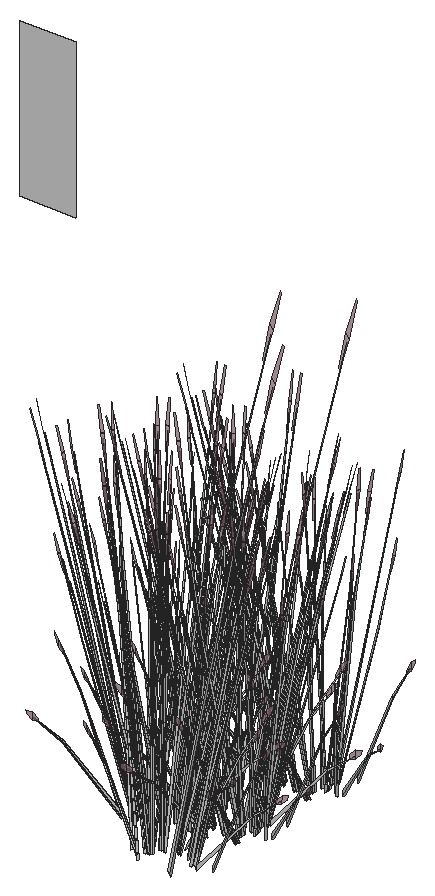
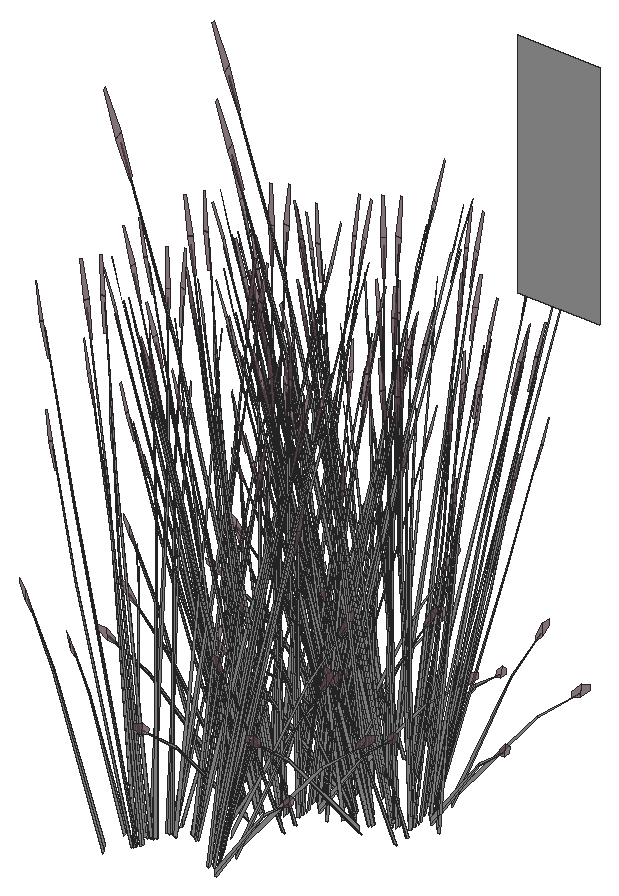
# SketchUp Ruby script. Lengths in inches.
U = 1.inch
M = Sketchup.active_model
def pt(a) = Geom::Point3d.new(a.map { |v| v * U })
def face(e, loops, mat)
  f = e.add_face(loops[0].map { |a| pt(a) })
  loops[1..].each { |l| e.add_face(l.map { |a| pt(a) }).erase! }
  f.material = f.back_material = mat if mat
  f
end
# faces: each face lists its corners as indices into pts; further lists are holes
def faces(e, pts, list, mat = nil) = list.each { |f| face(e, (f[0].is_a?(Array) ? f : [f]).map { |l| l.map { |i| pts[i] } }, mat) }
# xy, xz, yz: faces in a plane at the given z, y or x. An outline is a flat list of corners, or four numbers for a rectangle; further outlines are holes
def ring(l) = l.size == 4 ? [[l[0], l[1]], [l[2], l[1]], [l[2], l[3]], [l[0], l[3]]] : l.each_slice(2).to_a
def flat(e, list, mat, &to3) = list.each { |f| face(e, (f[0].is_a?(Array) ? f : [f]).map { |l| ring(l).map { |u, v| to3.(u, v) } }, mat) }
def xy(e, z, list, mat = nil) = flat(e, list, mat) { |x, y| [x, y, z] }
def xz(e, y, list, mat = nil) = flat(e, list, mat) { |x, z| [x, y, z] }
def yz(e, x, list, mat = nil) = flat(e, list, mat) { |y, z| [x, y, z] }
def lines(e, pts, list) = list.each { |a, b| e.add_line(pt(pts[a]), pt(pts[b])) }
# prism: a flat outline (further loops are holes) pulled along v
def prism(e, loops, v, mat = nil)
  f = face(e, loops, mat); d = Geom::Vector3d.new(v.map { |x| x * U })
  f.pushpull(f.normal.samedirection?(d) ? d.length : -d.length)
end
def box(e, o, s, mat = nil) = prism(e, [[o, [o[0] + s[0], o[1], o[2]], [o[0] + s[0], o[1] + s[1], o[2]], [o[0], o[1] + s[1], o[2]]]], [0, 0, s[2]], mat)
def at(x, y, z, deg = 0) = Geom::Transformation.translation(pt([x, y, z])) * Geom::Transformation.rotation(ORIGIN, Z_AXIS, deg.degrees)
def axes(o, x, y, z) = Geom::Transformation.new([*x, 0, *y, 0, *z, 0, *pt(o).to_a, 1])
def part(name) = M.definitions.add(name)
# library, detail: a bought-in or finely detailed component or shape, given as its bounding box
def library(name, o, s) = part(name).tap { |d| box(d.entities, o, s) }
def detail(e, o, s) = box(e.add_group.entities, o, s)
def put(e, d, t, mat = nil) = e.add_instance(d, t).tap { |i| i.material = mat if mat }
def group(e, t, mat = nil) = e.add_group.tap { |g| g.transformation = t; g.material = mat if mat }.entities
root = M.entities
M.materials.add("LightPink_Translucent").color = [144, 107, 117]
M.materials["LightPink_Translucent"].alpha = 0.75
M.materials.add("[_0053_Ivory_]").color = [200, 200, 200]
c1 = part("blade")
p = [[2.15,0.21,22],[0,0.17,0],[0.09,0.45,0],[2.18,0.31,22],[2.29,0.31,22],[0.38,0.45,0],
  [2.48,0.24,33],[2.49,0.24,33],[2.48,0.22,33]]
faces(c1.entities,p,[[0,1,2,3],[4,5,2,3],[6,3,4,7],[8,0,3,6]])
c2 = part("seeds")
p = [[0.3,-0.1,1.38],[-0.01,-0.03,1.59],[-0.01,-0.03,0.03],[0.14,-0.07,-0.07],[0.29,-0.03,3],[0.15,0.01,3.11]]
faces(c2.entities,p,[[0,1,2,3],[1,0,4,5]],"LightPink_Translucent")
c3 = part("blade with seeds")
put(c3.entities,c1,at(0,0,0))
put(c3.entities,c2,axes([2.4,0.25,30.99],[1.5799,-0.05474,1.17369],[-0.12525,1.92788,0.29478],[-0.07173,-0.02425,1.56792]))
xz(root,332.15,[[647.1,87,653.51,105]],"[_0053_Ivory_]")
put(root,c3,axes([674.04,316.75,38.39],[0.59846,0.1644,0.48003],[-0.20464,0.54049,0.3958],[-0.03596,-0.21255,0.9933]),"[_0053_Ivory_]")
put(root,c3,axes([674.21,316.94,38.6875],[-0.59433,0.29278,-0.1216],[-0.29207,-0.51964,-0.67495],[-0.07842,-0.21898,1.02557]),"[_0053_Ivory_]")
put(root,c3,axes([675.45,317.6,38.6875],[-0.6675,-0.03116,-0.1216],[0.01824,-0.58993,-0.67495],[0.04637,-0.2272,1.02557]),"[_0053_Ivory_]")
put(root,c3,axes([674.2,316.71,38.38],[0.44753,-0.21372,0.0643],[0.21905,0.38973,0.50621],[-0.04322,-0.1718,0.77189]),"[_0053_Ivory_]")
put(root,c3,axes([683.6875,314.28,38.36],[-0.05492,-0.05505,1.77383],[0.12013,-0.59013,-0.16761],[0.21632,-0.0377,0.31391]),"[_0053_Ivory_]")
put(root,c3,axes([676.54,311.89,38.37],[-0.09918,0.08165,1.74944],[0.00844,0.59653,-0.27667],[-0.22734,0.07758,0.14031]),"[_0053_Ivory_]")
put(root,c3,axes([677.18,311.32,38.6875],[0.30559,0.56943,-0.1216],[-0.54237,0.27983,-0.67495],[-0.22856,0.07513,1.02557]),"[_0053_Ivory_]")
put(root,c3,axes([681.79,313.77,38.6875],[0.03252,-0.63953,-0.1216],[0.61574,0.01748,-0.67495],[0.23714,0.04442,1.02557]),"[_0053_Ivory_]")
put(root,c3,axes([681.69,313.52,38.7],[-0.34557,-0.39372,0.35414],[0.39459,-0.37271,-0.4572],[0.20048,0.05671,0.87481]),"[_0053_Ivory_]")
put(root,c3,axes([672.67,316.77,38.38],[0.27604,-0.39948,0.0643],[0.39309,0.23258,0.50621],[-0.12709,-0.12808,0.77189]),"[_0053_Ivory_]")
put(root,c3,axes([674.03,317.15,38.7],[-0.1831,0.48359,0.35414],[-0.53419,-0.14105,-0.4572],[-0.04898,-0.1947,0.87481]),"[_0053_Ivory_]")
put(root,c3,axes([675.4,317.35,38.39],[0.43249,0.42907,0.48003],[-0.45929,0.37004,0.3958],[0.07978,-0.2013,0.9933]),"[_0053_Ivory_]")
put(root,c3,axes([672.79,316.73,39.08],[-0.40534,0.60286,-0.13619],[-0.58702,-0.34732,-0.75594],[-0.20405,-0.17032,1.14864]),"[_0053_Ivory_]")
put(root,c3,axes([682.32,313.39,38.37],[0.13029,-0.01064,1.74944],[0.35737,-0.48855,-0.27667],[0.23175,0.06449,0.14031]),"[_0053_Ivory_]")
put(root,c3,axes([675.56,317.39,38.38],[0.49911,0.0293,0.0643],[-0.01368,0.44245,0.50621],[0.05223,-0.16948,0.77189]),"[_0053_Ivory_]")
put(root,c3,axes([677.11,312.91,38.39],[-0.15063,-0.57876,0.48003],[0.59087,-0.10045,0.3958],[-0.17414,0.13612,0.9933]),"[_0053_Ivory_]")
put(root,c3,axes([677,312.8,38.38],[-0.41695,-0.26447,0.0643],[0.24275,-0.37662,0.50621],[-0.13368,0.12176,0.77189]),"[_0053_Ivory_]")
put(root,c3,axes([675.1875,317.69,38.7],[-0.41095,0.33109,0.35414],[-0.38901,-0.37805,-0.4572],[0.05919,-0.19208,0.87481]),"[_0053_Ivory_]")
put(root,c3,axes([679.55,318.65,38.37],[-0.0929,-0.08817,1.74944],[-0.61994,0.0559,-0.27667],[-0.09894,-0.21089,0.14031]),"[_0053_Ivory_]")
put(root,c3,axes([671.24,316.55,38.37],[-0.13068,-0.00444,1.74944],[-0.41604,0.44388,-0.27667],[-0.22198,-0.0907,0.14031]),"[_0053_Ivory_]")
put(root,c3,axes([676.17,318.76,38.6875],[-0.56181,-0.34675,-0.1216],[0.32367,-0.50216,-0.67495],[0.15873,-0.17455,1.02557]),"[_0053_Ivory_]")
put(root,c3,axes([677.48,312.72,38.7],[0.52868,-0.08987,0.35414],[0.1396,0.51376,-0.4572],[-0.1515,0.13799,0.87481]),"[_0053_Ivory_]")
put(root,c3,axes([675.4375,312.49,38.36],[0.07751,0.01687,1.77383],[0.23978,0.55562,-0.16761],[-0.15867,0.14583,0.31391]),"[_0053_Ivory_]")
put(root,c3,axes([672.75,317.23,38.7],[0.0938,0.50652,0.35414],[-0.53623,0.13375,-0.4572],[-0.14403,-0.14515,0.87481]),"[_0053_Ivory_]")
put(root,c3,axes([671.14,317.56,38.75],[0.50157,-0.46409,0.53763],[0.43258,0.49285,0.4433],[-0.23532,-0.08561,1.11249]),"[_0053_Ivory_]")
put(root,c3,axes([677.56,318.61,38.36],[-0.07933,-0.00478,1.77383],[-0.32942,-0.51175,-0.16761],[0.13229,-0.16826,0.31391]),"[_0053_Ivory_]")
put(root,c3,axes([682.01,313.88,38.38],[-0.03058,0.47819,0.0643],[-0.4618,-0.01311,0.50621],[0.1769,0.05004,0.77189]),"[_0053_Ivory_]")
put(root,c3,axes([682.33,319.73,38.37],[-0.00586,-0.12516,1.74944],[-0.49517,-0.36172,-0.27667],[0.07656,-0.21927,0.14031]),"[_0053_Ivory_]")
put(root,c3,axes([682.2,319.28,38.36],[-0.06168,0.04803,1.77383],[-0.60432,-0.16205,-0.16761],[-0.02188,-0.20961,0.31391]),"[_0053_Ivory_]")
put(root,c3,axes([682.05,313.73,38.39],[-0.44783,0.41436,0.48003],[-0.38623,-0.44004,0.3958],[0.21011,0.07643,0.9933]),"[_0053_Ivory_]")
put(root,c3,axes([676.28,314.18,39.3],[0.53595,0.16786,-0.06488],[-0.16486,0.51664,-0.29416],[-0.08766,0.07844,0.97024]),"[_0053_Ivory_]")
put(root,c3,axes([671.37,317.55,38.38],[0.03058,-0.47819,0.0643],[0.4618,0.01311,0.50621],[-0.1769,-0.05004,0.77189]),"[_0053_Ivory_]")
put(root,c3,axes([678.91,318.36,38.36],[-0.01133,0.07538,1.77383],[-0.55883,0.27355,-0.16761],[-0.16445,-0.13983,0.31391]),"[_0053_Ivory_]")
put(root,c3,axes([680.625,314.21,38.7],[-0.0938,-0.50652,0.35414],[0.53623,-0.13375,-0.4572],[0.14403,0.14515,0.87481]),"[_0053_Ivory_]")
put(root,c3,axes([678.79,319.7,38.75],[0.67657,-0.16163,0.53763],[0.11742,0.63404,0.4433],[-0.15912,-0.18687,1.11249]),"[_0053_Ivory_]")
put(root,c3,axes([675.9,318.71,38.7],[-0.52868,0.08987,0.35414],[-0.1396,-0.51376,-0.4572],[0.1515,-0.13799,0.87481]),"[_0053_Ivory_]")
put(root,c3,axes([680.98,311.29,38.13],[-0.52482,-0.32674,1.38283],[0.55416,-0.50872,0.59665],[0.16933,0.30658,1.33663]),"[_0053_Ivory_]")
put(root,c3,axes([680.32,319.82,38.39],[0.59846,0.1644,0.48003],[-0.20464,0.54049,0.3958],[-0.03596,-0.21255,0.9933]),"[_0053_Ivory_]")
put(root,c3,axes([680.49,320.01,38.6875],[-0.59433,0.29278,-0.1216],[-0.29207,-0.51964,-0.67495],[-0.07842,-0.21898,1.02557]),"[_0053_Ivory_]")
put(root,c3,axes([681.72,320.67,38.6875],[-0.6675,-0.03116,-0.1216],[0.01824,-0.58993,-0.67495],[0.04637,-0.2272,1.02557]),"[_0053_Ivory_]")
put(root,c3,axes([677.2,312.67,38.6875],[0.56181,0.34675,-0.1216],[-0.32367,0.50216,-0.67495],[-0.15873,0.17455,1.02557]),"[_0053_Ivory_]")
put(root,c3,axes([680.48,319.78,38.38],[0.44753,-0.21372,0.0643],[0.21905,0.38973,0.50621],[-0.04322,-0.1718,0.77189]),"[_0053_Ivory_]")
put(root,c3,axes([680.57,314.47,38.6875],[0.36191,-0.53827,-0.1216],[0.52412,0.3101,-0.67495],[0.18219,0.15207,1.02557]),"[_0053_Ivory_]")
put(root,c3,axes([678.1875,313.74,38.7],[0.41095,-0.33109,0.35414],[0.38901,0.37805,-0.4572],[-0.05919,0.19208,0.87481]),"[_0053_Ivory_]")
put(root,c3,axes([676.38,318.63,38.38],[0.41695,0.26447,0.0643],[-0.24275,0.37662,0.50621],[0.13368,-0.12176,0.77189]),"[_0053_Ivory_]")
put(root,c3,axes([680.1,314.91,38.36],[0.0018,-0.07613,1.77383],[0.52048,-0.3359,-0.16761],[0.18079,0.11989,0.31391]),"[_0053_Ivory_]")
put(root,c3,axes([676.26,318.52,38.39],[0.15063,0.57876,0.48003],[-0.59087,0.10045,0.3958],[0.17414,-0.13612,0.9933]),"[_0053_Ivory_]")
put(root,c3,axes([677.86,319.22,38.37],[0.08428,-0.09579,1.74944],[-0.10787,-0.58756,-0.27667],[0.21147,-0.1114,0.14031]),"[_0053_Ivory_]")
put(root,c3,axes([677.82,314.04,38.38],[-0.49911,-0.0293,0.0643],[0.01368,-0.44245,0.50621],[-0.05223,0.16948,0.77189]),"[_0053_Ivory_]")
put(root,c3,axes([678.94,319.83,38.38],[0.27604,-0.39948,0.0643],[0.39309,0.23258,0.50621],[-0.12709,-0.12808,0.77189]),"[_0053_Ivory_]")
put(root,c3,axes([677.98,314.08,38.39],[-0.43249,-0.42907,0.48003],[0.45929,-0.37004,0.3958],[-0.07978,0.2013,0.9933]),"[_0053_Ivory_]")
put(root,c3,axes([679.34,314.29,38.7],[0.1831,-0.48359,0.35414],[0.53419,0.14105,-0.4572],[0.04898,0.1947,0.87481]),"[_0053_Ivory_]")
put(root,c3,axes([670.73,316.93,38.36],[0.04503,0.06276,1.77383],[-0.21706,0.56413,-0.16761],[-0.21983,0.00408,0.31391]),"[_0053_Ivory_]")
put(root,c3,axes([680.31,320.21,38.7],[-0.1831,0.48359,0.35414],[-0.53419,-0.14105,-0.4572],[-0.04898,-0.1947,0.87481]),"[_0053_Ivory_]")
put(root,c3,axes([681.68,320.42,38.39],[0.43249,0.42907,0.48003],[-0.45929,0.37004,0.3958],[0.07978,-0.2013,0.9933]),"[_0053_Ivory_]")
put(root,c3,axes([679.07,319.79,39.08],[-0.40534,0.60286,-0.13619],[-0.58702,-0.34732,-0.75594],[-0.20405,-0.17032,1.14864]),"[_0053_Ivory_]")
put(root,c3,axes([680.71,314.66,38.38],[-0.27604,0.39948,0.0643],[-0.39309,-0.23258,0.50621],[0.12709,0.12808,0.77189]),"[_0053_Ivory_]")
put(root,c3,axes([681.84,320.46,38.38],[0.49911,0.0293,0.0643],[-0.01368,0.44245,0.50621],[0.05223,-0.16948,0.77189]),"[_0053_Ivory_]")
put(root,c3,axes([671.68,317.91,38.7],[0.34557,0.39372,0.35414],[-0.39459,0.37271,-0.4572],[-0.20048,-0.05671,0.87481]),"[_0053_Ivory_]")
put(root,c3,axes([680.06,316.01,39.3],[0.4197,-0.36076,-0.06488],[0.38456,0.39511,-0.29416],[0.02707,0.11196,0.97024]),"[_0053_Ivory_]")
put(root,c3,axes([680.82,314.55,38.39],[-0.60408,0.14432,0.48003],[-0.10484,-0.56611,0.3958],[0.14207,0.16684,0.9933]),"[_0053_Ivory_]")
put(root,c3,axes([681.46,320.76,38.7],[-0.41095,0.33109,0.35414],[-0.38901,-0.37805,-0.4572],[0.05919,-0.19208,0.87481]),"[_0053_Ivory_]")
put(root,c3,axes([671.59,317.66,38.6875],[-0.03252,0.63953,-0.1216],[-0.61574,-0.01748,-0.67495],[-0.23714,-0.04442,1.02557]),"[_0053_Ivory_]")
put(root,c3,axes([676.2,320.11,38.6875],[-0.30559,-0.56943,-0.1216],[0.54237,-0.27983,-0.67495],[0.22856,-0.07513,1.02557]),"[_0053_Ivory_]")
put(root,c3,axes([679.18,314.72,38.38],[-0.44753,0.21372,0.0643],[-0.21905,-0.38973,0.50621],[0.04322,0.1718,0.77189]),"[_0053_Ivory_]")
put(root,c3,axes([677.51,319.62,38.37],[-0.13068,-0.00444,1.74944],[-0.41604,0.44388,-0.27667],[-0.22198,-0.0907,0.14031]),"[_0053_Ivory_]")
put(root,c3,axes([682.45,321.83,38.6875],[-0.56181,-0.34675,-0.1216],[0.32367,-0.50216,-0.67495],[0.15873,-0.17455,1.02557]),"[_0053_Ivory_]")
put(root,c3,axes([676.56,314.11,38.37],[-0.0151,0.12444,1.74944],[0.42844,0.43292,-0.27667],[-0.11216,0.20472,0.14031]),"[_0053_Ivory_]")
put(root,c3,axes([677.93,313.83,39.05],[0.6675,0.03116,-0.13498],[-0.01824,0.58993,-0.74919],[-0.04637,0.2272,1.13838]),"[_0053_Ivory_]")
put(root,c3,axes([679.16,314.49,38.6875],[0.59433,-0.29278,-0.1216],[0.29207,0.51964,-0.67495],[0.07842,0.21898,1.02557]),"[_0053_Ivory_]")
put(root,c3,axes([679.33,314.68,38.72],[-0.59846,-0.1644,0.53283],[0.20464,-0.54049,0.43934],[0.03596,0.21255,1.10256]),"[_0053_Ivory_]")
put(root,c3,axes([679.03,320.29,38.7],[0.0938,0.50652,0.35414],[-0.53623,0.13375,-0.4572],[-0.14403,-0.14515,0.87481]),"[_0053_Ivory_]")
put(root,c3,axes([677.42,320.625,38.75],[0.50157,-0.46409,0.53763],[0.43258,0.49285,0.4433],[-0.23532,-0.08561,1.11249]),"[_0053_Ivory_]")
put(root,c3,axes([683.83,321.68,38.36],[-0.07933,-0.00478,1.77383],[-0.32942,-0.51175,-0.16761],[0.13229,-0.16826,0.31391]),"[_0053_Ivory_]")
put(root,c3,axes([675.98,319.94,38.7],[-0.50475,-0.17543,0.35414],[0.14722,-0.5118,-0.4572],[0.20322,-0.04693,0.87481]),"[_0053_Ivory_]")
put(root,c3,axes([670.7,319.01,38.39],[0.17159,-0.57338,0.48003],[0.56413,0.19607,0.3958],[-0.22185,0.03446,0.9933]),"[_0053_Ivory_]")
put(root,c3,axes([670.66,318.86,38.38],[-0.22307,-0.42878,0.0643],[0.40677,-0.20987,0.50621],[-0.17931,0.04141,0.77189]),"[_0053_Ivory_]")
put(root,c3,axes([677.65,320.62,38.38],[0.03058,-0.47819,0.0643],[0.4618,0.01311,0.50621],[-0.1769,-0.05004,0.77189]),"[_0053_Ivory_]")
put(root,c3,axes([676.51,315.39,38.36],[0.0689,-0.03797,1.77383],[0.5695,0.25254,-0.16761],[-0.01338,0.21027,0.31391]),"[_0053_Ivory_]")
put(root,c3,axes([682.18,321.78,38.7],[-0.52868,0.08987,0.35414],[-0.1396,-0.51376,-0.4572],[0.1515,-0.13799,0.87481]),"[_0053_Ivory_]")
put(root,c3,axes([679.02,315.65,38.37],[0.07699,0.10127,1.74944],[0.6213,0.03978,-0.27667],[0.06248,0.22333,0.14031]),"[_0053_Ivory_]")
put(root,c3,axes([682.66,321.7,38.38],[0.41695,0.26447,0.0643],[-0.24275,0.37662,0.50621],[0.13368,-0.12176,0.77189]),"[_0053_Ivory_]")
put(root,c3,axes([682.54,321.59,38.39],[0.15063,0.57876,0.48003],[-0.59087,0.10045,0.3958],[0.17414,-0.13612,0.9933]),"[_0053_Ivory_]")
put(root,c3,axes([684.13,322.29,38.37],[0.08428,-0.09579,1.74944],[-0.10787,-0.58756,-0.27667],[0.21147,-0.1114,0.14031]),"[_0053_Ivory_]")
put(root,c3,axes([676.44,320.1,38.38],[0.22307,0.42878,0.0643],[-0.40677,0.20987,0.50621],[0.17931,-0.04141,0.77189]),"[_0053_Ivory_]")
put(root,c3,axes([676.4,319.95,38.39],[-0.17159,0.57338,0.48003],[-0.56413,-0.19607,0.3958],[0.22185,-0.03446,0.9933]),"[_0053_Ivory_]")
put(root,c3,axes([671.12,319.01,38.7],[0.50475,0.17543,0.35414],[-0.14722,0.5118,-0.4572],[-0.20322,0.04693,0.87481]),"[_0053_Ivory_]")
put(root,c3,axes([677.01,320,38.36],[0.04503,0.06276,1.77383],[-0.21706,0.56413,-0.16761],[-0.21983,0.00408,0.31391]),"[_0053_Ivory_]")
put(root,c3,axes([677.96,320.98,38.7],[0.34557,0.39372,0.35414],[-0.39459,0.37271,-0.4572],[-0.20048,-0.05671,0.87481]),"[_0053_Ivory_]")
put(root,c3,axes([677.87,320.73,38.6875],[-0.03252,0.63953,-0.1216],[-0.61574,-0.01748,-0.67495],[-0.23714,-0.04442,1.02557]),"[_0053_Ivory_]")
put(root,c3,axes([677.41,321.81,38.36],[-0.05492,-0.05505,1.77383],[0.12013,-0.59013,-0.16761],[0.21632,-0.0377,0.31391]),"[_0053_Ivory_]")
put(root,c3,axes([682.47,323.18,38.6875],[-0.30559,-0.56943,-0.1216],[0.54237,-0.27983,-0.67495],[0.22856,-0.07513,1.02557]),"[_0053_Ivory_]")
put(root,c3,axes([670.26,319.41,38.37],[-0.09918,0.08165,1.74944],[0.00844,0.59653,-0.27667],[-0.22734,0.07758,0.14031]),"[_0053_Ivory_]")
put(root,c3,axes([670.9,318.84,38.6875],[0.30559,0.56943,-0.1216],[-0.54237,0.27983,-0.67495],[-0.22856,0.07513,1.02557]),"[_0053_Ivory_]")
put(root,c3,axes([675.51,321.3,38.6875],[0.03252,-0.63953,-0.1216],[0.61574,0.01748,-0.67495],[0.23714,0.04442,1.02557]),"[_0053_Ivory_]")
put(root,c3,axes([675.42,321.05,38.7],[-0.34557,-0.39372,0.35414],[0.39459,-0.37271,-0.4572],[0.20048,0.05671,0.87481]),"[_0053_Ivory_]")
put(root,c3,axes([682.26,323.01,38.7],[-0.50475,-0.17543,0.35414],[0.14722,-0.5118,-0.4572],[0.20322,-0.04693,0.87481]),"[_0053_Ivory_]")
put(root,c3,axes([676.98,322.08,38.39],[0.17159,-0.57338,0.48003],[0.56413,0.19607,0.3958],[-0.22185,0.03446,0.9933]),"[_0053_Ivory_]")
put(root,c3,axes([676.05,320.91,38.37],[0.13029,-0.01064,1.74944],[0.35737,-0.48855,-0.27667],[0.23175,0.06449,0.14031]),"[_0053_Ivory_]")
put(root,c3,axes([676.93,321.92,38.38],[-0.22307,-0.42878,0.0643],[0.40677,-0.20987,0.50621],[-0.17931,0.04141,0.77189]),"[_0053_Ivory_]")
put(root,c3,axes([670.84,320.44,38.39],[-0.15063,-0.57876,0.48003],[0.59087,-0.10045,0.3958],[-0.17414,0.13612,0.9933]),"[_0053_Ivory_]")
put(root,c3,axes([670.72,320.32,38.38],[-0.41695,-0.26447,0.0643],[0.24275,-0.37662,0.50621],[-0.13368,0.12176,0.77189]),"[_0053_Ivory_]")
put(root,c3,axes([671.2,320.24,38.7],[0.52868,-0.08987,0.35414],[0.1396,0.51376,-0.4572],[-0.1515,0.13799,0.87481]),"[_0053_Ivory_]")
put(root,c3,axes([669.16,320.01,38.36],[0.07751,0.01687,1.77383],[0.23978,0.55562,-0.16761],[-0.15867,0.14583,0.31391]),"[_0053_Ivory_]")
put(root,c3,axes([675.73,321.4,38.38],[-0.03058,0.47819,0.0643],[-0.4618,-0.01311,0.50621],[0.1769,0.05004,0.77189]),"[_0053_Ivory_]")
put(root,c3,axes([682.72,323.17,38.38],[0.22307,0.42878,0.0643],[-0.40677,0.20987,0.50621],[0.17931,-0.04141,0.77189]),"[_0053_Ivory_]")
put(root,c3,axes([675.77,321.25,38.39],[-0.44783,0.41436,0.48003],[-0.38623,-0.44004,0.3958],[0.21011,0.07643,0.9933]),"[_0053_Ivory_]")
put(root,c3,axes([682.68,323.02,38.39],[-0.17159,0.57338,0.48003],[-0.56413,-0.19607,0.3958],[0.22185,-0.03446,0.9933]),"[_0053_Ivory_]")
put(root,c3,axes([677.39,322.08,38.7],[0.50475,0.17543,0.35414],[-0.14722,0.5118,-0.4572],[-0.20322,0.04693,0.87481]),"[_0053_Ivory_]")
put(root,c3,axes([670,321.7,39.3],[0.53595,0.16786,-0.06488],[-0.16486,0.51664,-0.29416],[-0.08766,0.07844,0.97024]),"[_0053_Ivory_]")
put(root,c3,axes([674.35,321.73,38.7],[-0.0938,-0.50652,0.35414],[0.53623,-0.13375,-0.4572],[0.14403,0.14515,0.87481]),"[_0053_Ivory_]")
put(root,c3,axes([674.71,318.82,38.13],[-0.52482,-0.32674,1.38283],[0.55416,-0.50872,0.59665],[0.16933,0.30658,1.33663]),"[_0053_Ivory_]")
put(root,c3,axes([670.93,320.2,38.6875],[0.56181,0.34675,-0.1216],[-0.32367,0.50216,-0.67495],[-0.15873,0.17455,1.02557]),"[_0053_Ivory_]")
put(root,c3,axes([683.6875,324.875,38.36],[-0.05492,-0.05505,1.77383],[0.12013,-0.59013,-0.16761],[0.21632,-0.0377,0.31391]),"[_0053_Ivory_]")
put(root,c3,axes([674.3,321.99,38.6875],[0.36191,-0.53827,-0.1216],[0.52412,0.3101,-0.67495],[0.18219,0.15207,1.02557]),"[_0053_Ivory_]")
put(root,c3,axes([676.54,322.48,38.37],[-0.09918,0.08165,1.74944],[0.00844,0.59653,-0.27667],[-0.22734,0.07758,0.14031]),"[_0053_Ivory_]")
put(root,c3,axes([677.18,321.91,38.6875],[0.30559,0.56943,-0.1216],[-0.54237,0.27983,-0.67495],[-0.22856,0.07513,1.02557]),"[_0053_Ivory_]")
put(root,c3,axes([681.79,324.36,38.6875],[0.03252,-0.63953,-0.1216],[0.61574,0.01748,-0.67495],[0.23714,0.04442,1.02557]),"[_0053_Ivory_]")
put(root,c3,axes([671.91,321.27,38.7],[0.41095,-0.33109,0.35414],[0.38901,0.37805,-0.4572],[-0.05919,0.19208,0.87481]),"[_0053_Ivory_]")
put(root,c3,axes([673.82,322.44,38.36],[0.0018,-0.07613,1.77383],[0.52048,-0.3359,-0.16761],[0.18079,0.11989,0.31391]),"[_0053_Ivory_]")
put(root,c3,axes([681.69,324.11,38.7],[-0.34557,-0.39372,0.35414],[0.39459,-0.37271,-0.4572],[0.20048,0.05671,0.87481]),"[_0053_Ivory_]")
put(root,c3,axes([671.54,321.57,38.38],[-0.49911,-0.0293,0.0643],[0.01368,-0.44245,0.50621],[-0.05223,0.16948,0.77189]),"[_0053_Ivory_]")
put(root,c3,axes([671.7,321.61,38.39],[-0.43249,-0.42907,0.48003],[0.45929,-0.37004,0.3958],[-0.07978,0.2013,0.9933]),"[_0053_Ivory_]")
put(root,c3,axes([673.07,321.8125,38.7],[0.1831,-0.48359,0.35414],[0.53419,0.14105,-0.4572],[0.04898,0.1947,0.87481]),"[_0053_Ivory_]")
put(root,c3,axes([679.55,328.79,38.37],[-0.0929,-0.08817,1.74944],[-0.61994,0.0559,-0.27667],[-0.09894,-0.21089,0.14031]),"[_0053_Ivory_]")
put(root,c3,axes([682.32,323.98,38.37],[0.13029,-0.01064,1.74944],[0.35737,-0.48855,-0.27667],[0.23175,0.06449,0.14031]),"[_0053_Ivory_]")
put(root,c3,axes([674.43,322.19,38.38],[-0.27604,0.39948,0.0643],[-0.39309,-0.23258,0.50621],[0.12709,0.12808,0.77189]),"[_0053_Ivory_]")
put(root,c3,axes([677.11,323.5,38.39],[-0.15063,-0.57876,0.48003],[0.59087,-0.10045,0.3958],[-0.17414,0.13612,0.9933]),"[_0053_Ivory_]")
put(root,c3,axes([673.78,323.54,39.3],[0.4197,-0.36076,-0.06488],[0.38456,0.39511,-0.29416],[0.02707,0.11196,0.97024]),"[_0053_Ivory_]")
put(root,c3,axes([677,323.39,38.38],[-0.41695,-0.26447,0.0643],[0.24275,-0.37662,0.50621],[-0.13368,0.12176,0.77189]),"[_0053_Ivory_]")
put(root,c3,axes([674.55,322.08,38.39],[-0.60408,0.14432,0.48003],[-0.10484,-0.56611,0.3958],[0.14207,0.16684,0.9933]),"[_0053_Ivory_]")
put(root,c3,axes([672.9,322.25,38.38],[-0.44753,0.21372,0.0643],[-0.21905,-0.38973,0.50621],[0.04322,0.1718,0.77189]),"[_0053_Ivory_]")
put(root,c3,axes([670.28,321.64,38.37],[-0.0151,0.12444,1.74944],[0.42844,0.43292,-0.27667],[-0.11216,0.20472,0.14031]),"[_0053_Ivory_]")
put(root,c3,axes([671.65,321.36,39.05],[0.6675,0.03116,-0.13498],[-0.01824,0.58993,-0.74919],[-0.04637,0.2272,1.13838]),"[_0053_Ivory_]")
put(root,c3,axes([682.33,329.87,38.37],[-0.00586,-0.12516,1.74944],[-0.49517,-0.36172,-0.27667],[0.07656,-0.21927,0.14031]),"[_0053_Ivory_]")
put(root,c3,axes([682.2,329.42,38.36],[-0.06168,0.04803,1.77383],[-0.60432,-0.16205,-0.16761],[-0.02188,-0.20961,0.31391]),"[_0053_Ivory_]")
put(root,c3,axes([672.89,322.01,38.6875],[0.59433,-0.29278,-0.1216],[0.29207,0.51964,-0.67495],[0.07842,0.21898,1.02557]),"[_0053_Ivory_]")
put(root,c3,axes([673.06,322.21,38.72],[-0.59846,-0.1644,0.53283],[0.20464,-0.54049,0.43934],[0.03596,0.21255,1.10256]),"[_0053_Ivory_]")
put(root,c3,axes([677.48,323.31,38.7],[0.52868,-0.08987,0.35414],[0.1396,0.51376,-0.4572],[-0.1515,0.13799,0.87481]),"[_0053_Ivory_]")
put(root,c3,axes([675.4375,323.08,38.36],[0.07751,0.01687,1.77383],[0.23978,0.55562,-0.16761],[-0.15867,0.14583,0.31391]),"[_0053_Ivory_]")
put(root,c3,axes([682.01,324.47,38.38],[-0.03058,0.47819,0.0643],[-0.4618,-0.01311,0.50621],[0.1769,0.05004,0.77189]),"[_0053_Ivory_]")
put(root,c3,axes([678.91,328.5,38.36],[-0.01133,0.07538,1.77383],[-0.55883,0.27355,-0.16761],[-0.16445,-0.13983,0.31391]),"[_0053_Ivory_]")
put(root,c3,axes([682.05,324.32,38.39],[-0.44783,0.41436,0.48003],[-0.38623,-0.44004,0.3958],[0.21011,0.07643,0.9933]),"[_0053_Ivory_]")
put(root,c3,axes([678.79,329.84,38.75],[0.67657,-0.16163,0.53763],[0.11742,0.63404,0.4433],[-0.15912,-0.18687,1.11249]),"[_0053_Ivory_]")
put(root,c3,axes([680.32,329.96,38.39],[0.59846,0.1644,0.48003],[-0.20464,0.54049,0.3958],[-0.03596,-0.21255,0.9933]),"[_0053_Ivory_]")
put(root,c3,axes([680.49,330.15,38.6875],[-0.59433,0.29278,-0.1216],[-0.29207,-0.51964,-0.67495],[-0.07842,-0.21898,1.02557]),"[_0053_Ivory_]")
put(root,c3,axes([681.72,330.81,38.6875],[-0.6675,-0.03116,-0.1216],[0.01824,-0.58993,-0.67495],[0.04637,-0.2272,1.02557]),"[_0053_Ivory_]")
put(root,c3,axes([676.28,324.77,39.3],[0.53595,0.16786,-0.06488],[-0.16486,0.51664,-0.29416],[-0.08766,0.07844,0.97024]),"[_0053_Ivory_]")
put(root,c3,axes([680.48,329.91,38.38],[0.44753,-0.21372,0.0643],[0.21905,0.38973,0.50621],[-0.04322,-0.1718,0.77189]),"[_0053_Ivory_]")
put(root,c3,axes([680.625,324.8,38.7],[-0.0938,-0.50652,0.35414],[0.53623,-0.13375,-0.4572],[0.14403,0.14515,0.87481]),"[_0053_Ivory_]")
put(root,c3,axes([670.23,322.91,38.36],[0.0689,-0.03797,1.77383],[0.5695,0.25254,-0.16761],[-0.01338,0.21027,0.31391]),"[_0053_Ivory_]")
put(root,c3,axes([680.98,321.88,38.13],[-0.52482,-0.32674,1.38283],[0.55416,-0.50872,0.59665],[0.16933,0.30658,1.33663]),"[_0053_Ivory_]")
put(root,c3,axes([677.2,323.26,38.6875],[0.56181,0.34675,-0.1216],[-0.32367,0.50216,-0.67495],[-0.15873,0.17455,1.02557]),"[_0053_Ivory_]")
put(root,c3,axes([680.57,325.0625,38.6875],[0.36191,-0.53827,-0.1216],[0.52412,0.3101,-0.67495],[0.18219,0.15207,1.02557]),"[_0053_Ivory_]")
put(root,c3,axes([678.94,329.97,38.38],[0.27604,-0.39948,0.0643],[0.39309,0.23258,0.50621],[-0.12709,-0.12808,0.77189]),"[_0053_Ivory_]")
put(root,c3,axes([672.75,323.18,38.37],[0.07699,0.10127,1.74944],[0.6213,0.03978,-0.27667],[0.06248,0.22333,0.14031]),"[_0053_Ivory_]")
put(root,c3,axes([678.1875,324.33,38.7],[0.41095,-0.33109,0.35414],[0.38901,0.37805,-0.4572],[-0.05919,0.19208,0.87481]),"[_0053_Ivory_]")
put(root,c3,axes([680.31,330.35,38.7],[-0.1831,0.48359,0.35414],[-0.53419,-0.14105,-0.4572],[-0.04898,-0.1947,0.87481]),"[_0053_Ivory_]")
put(root,c3,axes([680.1,325.51,38.36],[0.0018,-0.07613,1.77383],[0.52048,-0.3359,-0.16761],[0.18079,0.11989,0.31391]),"[_0053_Ivory_]")
put(root,c3,axes([677.82,324.63,38.38],[-0.49911,-0.0293,0.0643],[0.01368,-0.44245,0.50621],[-0.05223,0.16948,0.77189]),"[_0053_Ivory_]")
put(root,c3,axes([681.68,330.56,38.39],[0.43249,0.42907,0.48003],[-0.45929,0.37004,0.3958],[0.07978,-0.2013,0.9933]),"[_0053_Ivory_]")
put(root,c3,axes([677.98,324.67,38.39],[-0.43249,-0.42907,0.48003],[0.45929,-0.37004,0.3958],[-0.07978,0.2013,0.9933]),"[_0053_Ivory_]")
put(root,c3,axes([679.07,329.93,39.08],[-0.40534,0.60286,-0.13619],[-0.58702,-0.34732,-0.75594],[-0.20405,-0.17032,1.14864]),"[_0053_Ivory_]")
put(root,c3,axes([681.84,330.6,38.38],[0.49911,0.0293,0.0643],[-0.01368,0.44245,0.50621],[0.05223,-0.16948,0.77189]),"[_0053_Ivory_]")
put(root,c3,axes([679.34,324.88,38.7],[0.1831,-0.48359,0.35414],[0.53419,0.14105,-0.4572],[0.04898,0.1947,0.87481]),"[_0053_Ivory_]")
put(root,c3,axes([681.46,330.9,38.7],[-0.41095,0.33109,0.35414],[-0.38901,-0.37805,-0.4572],[0.05919,-0.19208,0.87481]),"[_0053_Ivory_]")
put(root,c3,axes([680.71,325.26,38.38],[-0.27604,0.39948,0.0643],[-0.39309,-0.23258,0.50621],[0.12709,0.12808,0.77189]),"[_0053_Ivory_]")
put(root,c3,axes([680.06,326.6,39.3],[0.4197,-0.36076,-0.06488],[0.38456,0.39511,-0.29416],[0.02707,0.11196,0.97024]),"[_0053_Ivory_]")
put(root,c3,axes([677.51,329.76,38.37],[-0.13068,-0.00444,1.74944],[-0.41604,0.44388,-0.27667],[-0.22198,-0.0907,0.14031]),"[_0053_Ivory_]")
put(root,c3,axes([682.45,331.97,38.6875],[-0.56181,-0.34675,-0.1216],[0.32367,-0.50216,-0.67495],[0.15873,-0.17455,1.02557]),"[_0053_Ivory_]")
put(root,c3,axes([680.82,325.15,38.39],[-0.60408,0.14432,0.48003],[-0.10484,-0.56611,0.3958],[0.14207,0.16684,0.9933]),"[_0053_Ivory_]")
put(root,c3,axes([679.03,330.43,38.7],[0.0938,0.50652,0.35414],[-0.53623,0.13375,-0.4572],[-0.14403,-0.14515,0.87481]),"[_0053_Ivory_]")
put(root,c3,axes([677.42,330.76,38.75],[0.50157,-0.46409,0.53763],[0.43258,0.49285,0.4433],[-0.23532,-0.08561,1.11249]),"[_0053_Ivory_]")
put(root,c3,axes([679.18,325.32,38.38],[-0.44753,0.21372,0.0643],[-0.21905,-0.38973,0.50621],[0.04322,0.1718,0.77189]),"[_0053_Ivory_]")
put(root,c3,axes([683.83,331.82,38.36],[-0.07933,-0.00478,1.77383],[-0.32942,-0.51175,-0.16761],[0.13229,-0.16826,0.31391]),"[_0053_Ivory_]")
put(root,c3,axes([676.56,324.71,38.37],[-0.0151,0.12444,1.74944],[0.42844,0.43292,-0.27667],[-0.11216,0.20472,0.14031]),"[_0053_Ivory_]")
put(root,c3,axes([677.93,324.42,39.05],[0.6675,0.03116,-0.13498],[-0.01824,0.58993,-0.74919],[-0.04637,0.2272,1.13838]),"[_0053_Ivory_]")
put(root,c3,axes([679.16,325.08,38.6875],[0.59433,-0.29278,-0.1216],[0.29207,0.51964,-0.67495],[0.07842,0.21898,1.02557]),"[_0053_Ivory_]")
put(root,c3,axes([679.33,325.28,38.72],[-0.59846,-0.1644,0.53283],[0.20464,-0.54049,0.43934],[0.03596,0.21255,1.10256]),"[_0053_Ivory_]")
put(root,c3,axes([677.65,330.76,38.38],[0.03058,-0.47819,0.0643],[0.4618,0.01311,0.50621],[-0.1769,-0.05004,0.77189]),"[_0053_Ivory_]")
put(root,c3,axes([682.18,331.92,38.7],[-0.52868,0.08987,0.35414],[-0.1396,-0.51376,-0.4572],[0.1515,-0.13799,0.87481]),"[_0053_Ivory_]")
put(root,c3,axes([676.51,325.98,38.36],[0.0689,-0.03797,1.77383],[0.5695,0.25254,-0.16761],[-0.01338,0.21027,0.31391]),"[_0053_Ivory_]")
put(root,c3,axes([682.66,331.84,38.38],[0.41695,0.26447,0.0643],[-0.24275,0.37662,0.50621],[0.13368,-0.12176,0.77189]),"[_0053_Ivory_]")
put(root,c3,axes([682.54,331.73,38.39],[0.15063,0.57876,0.48003],[-0.59087,0.10045,0.3958],[0.17414,-0.13612,0.9933]),"[_0053_Ivory_]")
put(root,c3,axes([684.13,332.43,38.37],[0.08428,-0.09579,1.74944],[-0.10787,-0.58756,-0.27667],[0.21147,-0.1114,0.14031]),"[_0053_Ivory_]")
put(root,c3,axes([677.01,330.14,38.36],[0.04503,0.06276,1.77383],[-0.21706,0.56413,-0.16761],[-0.21983,0.00408,0.31391]),"[_0053_Ivory_]")
put(root,c3,axes([679.02,326.25,38.37],[0.07699,0.10127,1.74944],[0.6213,0.03978,-0.27667],[0.06248,0.22333,0.14031]),"[_0053_Ivory_]")
put(root,c3,axes([677.96,331.12,38.7],[0.34557,0.39372,0.35414],[-0.39459,0.37271,-0.4572],[-0.20048,-0.05671,0.87481]),"[_0053_Ivory_]")
put(root,c3,axes([677.87,330.87,38.6875],[-0.03252,0.63953,-0.1216],[-0.61574,-0.01748,-0.67495],[-0.23714,-0.04442,1.02557]),"[_0053_Ivory_]")
put(root,c3,axes([682.47,333.32,38.6875],[-0.30559,-0.56943,-0.1216],[0.54237,-0.27983,-0.67495],[0.22856,-0.07513,1.02557]),"[_0053_Ivory_]")
put(root,c3,axes([682.26,333.15,38.7],[-0.50475,-0.17543,0.35414],[0.14722,-0.5118,-0.4572],[0.20322,-0.04693,0.87481]),"[_0053_Ivory_]")
put(root,c3,axes([676.98,332.21,38.39],[0.17159,-0.57338,0.48003],[0.56413,0.19607,0.3958],[-0.22185,0.03446,0.9933]),"[_0053_Ivory_]")
put(root,c3,axes([676.93,332.0625,38.38],[-0.22307,-0.42878,0.0643],[0.40677,-0.20987,0.50621],[-0.17931,0.04141,0.77189]),"[_0053_Ivory_]")
put(root,c3,axes([682.72,333.31,38.38],[0.22307,0.42878,0.0643],[-0.40677,0.20987,0.50621],[0.17931,-0.04141,0.77189]),"[_0053_Ivory_]")
put(root,c3,axes([682.68,333.16,38.39],[-0.17159,0.57338,0.48003],[-0.56413,-0.19607,0.3958],[0.22185,-0.03446,0.9933]),"[_0053_Ivory_]")
put(root,c3,axes([677.39,332.22,38.7],[0.50475,0.17543,0.35414],[-0.14722,0.5118,-0.4572],[-0.20322,0.04693,0.87481]),"[_0053_Ivory_]")
put(root,c3,axes([683.6875,335.01,38.36],[-0.05492,-0.05505,1.77383],[0.12013,-0.59013,-0.16761],[0.21632,-0.0377,0.31391]),"[_0053_Ivory_]")
put(root,c3,axes([676.54,332.62,38.37],[-0.09918,0.08165,1.74944],[0.00844,0.59653,-0.27667],[-0.22734,0.07758,0.14031]),"[_0053_Ivory_]")
